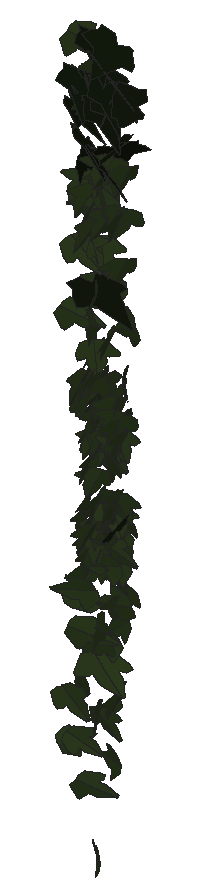
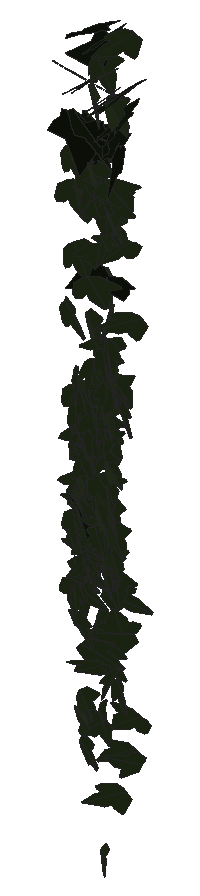
# SketchUp Ruby script. Lengths in inches.
U = 1.inch
M = Sketchup.active_model
def pt(a) = Geom::Point3d.new(a.map { |v| v * U })
def face(e, loops, mat)
  f = e.add_face(loops[0].map { |a| pt(a) })
  loops[1..].each { |l| e.add_face(l.map { |a| pt(a) }).erase! }
  f.material = f.back_material = mat if mat
  f
end
# faces: each face lists its corners as indices into pts; further lists are holes
def faces(e, pts, list, mat = nil) = list.each { |f| face(e, (f[0].is_a?(Array) ? f : [f]).map { |l| l.map { |i| pts[i] } }, mat) }
# xy, xz, yz: faces in a plane at the given z, y or x. An outline is a flat list of corners, or four numbers for a rectangle; further outlines are holes
def ring(l) = l.size == 4 ? [[l[0], l[1]], [l[2], l[1]], [l[2], l[3]], [l[0], l[3]]] : l.each_slice(2).to_a
def flat(e, list, mat, &to3) = list.each { |f| face(e, (f[0].is_a?(Array) ? f : [f]).map { |l| ring(l).map { |u, v| to3.(u, v) } }, mat) }
def xy(e, z, list, mat = nil) = flat(e, list, mat) { |x, y| [x, y, z] }
def xz(e, y, list, mat = nil) = flat(e, list, mat) { |x, z| [x, y, z] }
def yz(e, x, list, mat = nil) = flat(e, list, mat) { |y, z| [x, y, z] }
def lines(e, pts, list) = list.each { |a, b| e.add_line(pt(pts[a]), pt(pts[b])) }
# prism: a flat outline (further loops are holes) pulled along v
def prism(e, loops, v, mat = nil)
  f = face(e, loops, mat); d = Geom::Vector3d.new(v.map { |x| x * U })
  f.pushpull(f.normal.samedirection?(d) ? d.length : -d.length)
end
def box(e, o, s, mat = nil) = prism(e, [[o, [o[0] + s[0], o[1], o[2]], [o[0] + s[0], o[1] + s[1], o[2]], [o[0], o[1] + s[1], o[2]]]], [0, 0, s[2]], mat)
def at(x, y, z, deg = 0) = Geom::Transformation.translation(pt([x, y, z])) * Geom::Transformation.rotation(ORIGIN, Z_AXIS, deg.degrees)
def axes(o, x, y, z) = Geom::Transformation.new([*x, 0, *y, 0, *z, 0, *pt(o).to_a, 1])
def part(name) = M.definitions.add(name)
# library, detail: a bought-in or finely detailed component or shape, given as its bounding box
def library(name, o, s) = part(name).tap { |d| box(d.entities, o, s) }
def detail(e, o, s) = box(e.add_group.entities, o, s)
def put(e, d, t, mat = nil) = e.add_instance(d, t).tap { |i| i.material = mat if mat }
def group(e, t, mat = nil) = e.add_group.tap { |g| g.transformation = t; g.material = mat if mat }.entities
root = M.entities
M.materials.add("1026 AP 7946 SUNNY SIDE UP").color = [254, 231, 186]
M.materials.add("efeu1").color = [18, 25, 13]
M.materials.add("efeu2").color = [43, 57, 29]
c1 = part("ivyleaf_10")
p = [[0,0.5,-0.03],[-0.0625,2.02,-0.43],[-0.19,2.01,-0.46],[-0.54,1.05,-0.29],[-0.52,0.625,-0.18],[-0.83,0.76,-0.28],
  [-1.16,0.64,-0.33],[-1.15,0.33,-0.24],[-0.77,-0.39,0.02],[-0.3,-0.51,0.16],[0.04,-0.48,0.23],[-0.02,2.01,-0.4375],
  [-0.06,2.01,-0.43],[0.04,-0.49,0.23],[0.67,-0.49,0.14],[1.38,0.36,-0.2],[1.375,0.51,-0.24],[0.81,0.65,-0.19],
  [0.62,0.59,-0.15],[0.6,1.09,-0.28],[0.5,1.23,-0.31]]
faces(c1.entities,p,[[0,1,2,3,4,5,6,7,8,9,10],[11,12,0,13,14,15,16,17,18,19,20]],"efeu2")
c2 = part("ivyleaf_9")
p = [[1.54,2.16,1.25],[1.36,2.04,1.19],[-0.21,0.99,0.68],[-0.71,1.11,0.82],[-0.85,0.86,0.67],[-0.8,0.17,0.21],
  [-0.9,-0.01,0.1],[-0.67,-0.16,-0.02],[-0.08,-0.08,-0.05],[-0.03,-0.6,-0.4],[0.65,-0.88,-0.66],[0.83,-0.6,-0.49],
  [1.29,-0.42,-0.43],[1.8125,-0.07,-0.26],[1.21,0.44,0.15]]
faces(c2.entities,p,[[0,1,2,3,4,5,6,7,8,9,10,11,12,13,14]],"efeu1")
put(root,c1,axes([101.61,213.03,262.17],[0.23176,-0.14926,-0.08076],[-0.02073,0.09254,-0.20877],[0.26367,0.13847,0.05457]),"1026 AP 7946 SUNNY SIDE UP")
put(root,c2,axes([101.46,212.75,266.26],[0.24733,-0.16671,-0.10642],[-0.08833,0.08731,-0.23493],[0.29464,0.16612,0.0189]),"1026 AP 7946 SUNNY SIDE UP")
put(root,c1,axes([101.72,212.88,264.88],[-0.23689,-0.12528,0.14324],[-0.06836,-0.15104,-0.18865],[0.28709,-0.13934,0.07327]),"1026 AP 7946 SUNNY SIDE UP")
put(root,c1,axes([101.56,212.82,257.06],[0.27559,0.10864,-0.05443],[0.05387,0.0457,0.21169],[0.1826,-0.17745,0.0197]),"1026 AP 7946 SUNNY SIDE UP")
put(root,c2,axes([101.4375,213.02,266.65],[0.15677,-0.22108,-0.05738],[0.00234,0.06006,-0.24812],[0.35801,0.09642,0.02675]),"1026 AP 7946 SUNNY SIDE UP")
put(root,c1,axes([101.66,212.85,258.75],[-0.00671,-0.20722,0.02512],[-0.00265,-0.02553,-0.21367],[0.32829,-0.00444,-0.00121]),"1026 AP 7946 SUNNY SIDE UP")
put(root,c1,axes([101.59,212.96,256.3],[-0.03619,0.20773,0.06893],[-0.01152,0.06532,-0.21493],[-0.34241,-0.02415,-0.00006]),"1026 AP 7946 SUNNY SIDE UP")
put(root,c1,axes([101.86,212.6,257.48],[0.12653,0.00961,-0.2148],[-0.32827,0.006,-0.08266],[0.00337,0.22346,0.01276]),"1026 AP 7946 SUNNY SIDE UP")
put(root,c1,axes([101.42,212.63,255.43],[0.23805,0.04509,0.1535],[0.22598,0.03846,-0.16248],[-0.09307,0.20872,-0.0019]),"1026 AP 7946 SUNNY SIDE UP")
put(root,c1,axes([101.71,212.68,261],[0.22148,-0.18425,-0.10021],[-0.08169,0.08134,-0.23832],[0.31647,0.14994,0.00861]),"1026 AP 7946 SUNNY SIDE UP")
put(root,c1,axes([101.48,212.56,254.57],[0.08927,0.03452,-0.19843],[0.22167,0.13218,0.06791],[0.21384,-0.15142,0.01244]),"1026 AP 7946 SUNNY SIDE UP")
put(root,c2,axes([101.71,212.67,265.42],[0.07925,-0.05546,-0.25307],[-0.28866,0.16293,-0.07585],[0.27036,0.19022,-0.0068]),"1026 AP 7946 SUNNY SIDE UP")
put(root,c2,axes([101.54,212.87,266.64],[-0.03684,-0.24323,0.06027],[0.00647,-0.06051,-0.25189],[0.39382,-0.02176,0.00978]),"1026 AP 7946 SUNNY SIDE UP")
put(root,c1,axes([101.8125,212.59,255.85],[-0.14739,0.09172,0.16047],[-0.22078,0.07265,-0.13113],[-0.1779,-0.16616,0.02979]),"1026 AP 7946 SUNNY SIDE UP")
put(root,c1,axes([101.69,212.86,266.33],[0.04286,-0.2374,0.08742],[0.00963,-0.08606,-0.24665],[0.39701,0.02771,-0.00346]),"1026 AP 7946 SUNNY SIDE UP")
put(root,c1,axes([101.66,212.73,261.29],[0.01328,-0.20034,0.1191],[0.05041,-0.11469,-0.20582],[0.3611,0.02338,0.02435]),"1026 AP 7946 SUNNY SIDE UP")
put(root,c1,axes([101.72,212.88,261.76],[0.09502,-0.19344,-0.10823],[-0.02668,0.10339,-0.20774],[0.34427,0.0614,0.01377]),"1026 AP 7946 SUNNY SIDE UP")
put(root,c1,axes([101.47,212.64,262.49],[-0.11051,-0.10361,-0.20119],[0.30628,0.06671,-0.10861],[0.1627,-0.19596,0.0678]),"1026 AP 7946 SUNNY SIDE UP")
put(root,c1,axes([101.53,212.71,267.55],[-0.09663,-0.15585,-0.20096],[0.26263,0.12254,-0.15505],[0.29037,-0.1627,0.07336]),"1026 AP 7946 SUNNY SIDE UP")
put(root,c1,axes([101.73,212.83,258.35],[-0.01414,-0.20729,0.01577],[-0.00333,-0.0164,-0.21384],[0.32696,-0.00913,-0.0015]),"1026 AP 7946 SUNNY SIDE UP")
put(root,c1,axes([101.78,212.85,264.69],[-0.11994,-0.1968,0.11635],[-0.02853,-0.11465,-0.21697],[0.35653,-0.07538,0.02178]),"1026 AP 7946 SUNNY SIDE UP")
put(root,c1,axes([101.78,212.81,261.52],[0.09506,-0.21581,-0.0587],[-0.03511,0.05161,-0.23046],[0.34872,0.06403,-0.0072]),"1026 AP 7946 SUNNY SIDE UP")
put(root,c1,axes([101.77,212.69,257.78],[-0.1154,-0.18957,0.00063],[0.00594,-0.00327,-0.20938],[0.29803,-0.07334,0.00441]),"1026 AP 7946 SUNNY SIDE UP")
put(root,c1,axes([101.75,212.85,264.41],[0.14658,-0.22174,0.02744],[0.00316,-0.02939,-0.24778],[0.3514,0.09276,-0.00922]),"1026 AP 7946 SUNNY SIDE UP")
put(root,c1,axes([101.78,212.84,259.39],[0.1442,-0.18895,-0.06129],[-0.01091,0.06128,-0.21505],[0.31079,0.08982,0.02089]),"1026 AP 7946 SUNNY SIDE UP")
put(root,c1,axes([101.79,212.73,259.11],[0.03543,-0.20794,-0.03637],[0.00319,0.03453,-0.21519],[0.33133,0.0219,0.00596]),"1026 AP 7946 SUNNY SIDE UP")
put(root,c1,axes([101.79,212.88,264.54],[-0.26299,-0.16813,-0.00818],[0.03619,-0.0131,-0.24297],[0.26211,-0.16689,0.02534]),"1026 AP 7946 SUNNY SIDE UP")
put(root,c1,axes([101.82,212.78,264.08],[0.00136,-0.19115,0.14714],[0.01173,-0.14382,-0.19769],[0.37604,0.00518,0.00563]),"1026 AP 7946 SUNNY SIDE UP")
put(root,c1,axes([101.81,212.75,258.69],[-0.00967,-0.17007,-0.1392],[0.02296,0.13358,-0.17436],[0.33983,-0.01386,0.00782]),"1026 AP 7946 SUNNY SIDE UP")
put(root,c1,axes([101.8,212.88,258.02],[0.07527,-0.20039,-0.01726],[0.01418,0.01818,-0.21173],[0.31574,0.04696,0.01362]),"1026 AP 7946 SUNNY SIDE UP")
put(root,c1,axes([101.85,212.83,260.89],[0.0404,-0.21738,-0.05823],[-0.02444,0.05379,-0.225],[0.35184,0.0287,-0.00894]),"1026 AP 7946 SUNNY SIDE UP")
put(root,c1,axes([101.79,212.81,261.22],[-0.11763,-0.18359,-0.11534],[0.07918,0.09916,-0.20349],[0.32785,-0.08982,0.00776]),"1026 AP 7946 SUNNY SIDE UP")
put(root,c1,axes([101.85,212.86,261.83],[-0.05054,-0.22068,-0.04146],[0.0033,0.03909,-0.22949],[0.35236,-0.03202,-0.00379]),"1026 AP 7946 SUNNY SIDE UP")
put(root,c1,axes([101.84,212.98,259.08],[0.06676,-0.20368,0.01444],[-0.00351,-0.01596,-0.21436],[0.32113,0.04217,-0.00534]),"1026 AP 7946 SUNNY SIDE UP")
put(root,c1,axes([101.85,212.72,258.15],[-0.00269,-0.20464,0.01488],[0.00056,-0.01561,-0.21092],[0.32271,-0.00168,0.00049]),"1026 AP 7946 SUNNY SIDE UP")
put(root,c1,axes([101.86,212.66,258.57],[-0.03395,-0.19711,0.06331],[0.00278,-0.06309,-0.20447],[0.32517,-0.02004,0.00836]),"1026 AP 7946 SUNNY SIDE UP")
put(root,c1,axes([101.65,212.55,254.74],[0.11584,0.10359,0.16632],[0.17773,0.11551,-0.12928],[-0.24273,0.13401,-0.01529]),"1026 AP 7946 SUNNY SIDE UP")
put(root,c1,axes([101.84,212.74,259.83],[0.06507,-0.19625,0.0755],[0.01914,-0.07347,-0.20703],[0.32947,0.04303,-0.00289]),"1026 AP 7946 SUNNY SIDE UP")
put(root,c1,axes([101.88,212.92,267.09],[-0.05804,-0.24494,0.0506],[-0.00831,-0.05028,-0.25547],[0.39316,-0.03722,0.00207]),"1026 AP 7946 SUNNY SIDE UP")
put(root,c1,axes([101.66,212.625,263.79],[0.21552,0.17038,0.13839],[0.15447,0.09166,-0.22411],[-0.30313,0.16784,-0.01581]),"1026 AP 7946 SUNNY SIDE UP")
put(root,c1,axes([101.98,212.56,258.14],[0.23237,-0.0268,0.15395],[-0.22153,0.05408,0.15368],[-0.08961,-0.20321,0.0193]),"1026 AP 7946 SUNNY SIDE UP")
put(root,c1,axes([101.87,212.6875,261.42],[0.15944,-0.20959,0.04832],[0.0155,-0.04859,-0.23982],[0.33777,0.10116,-0.0118]),"1026 AP 7946 SUNNY SIDE UP")
put(root,c1,axes([101.98,212.74,256.53],[-0.30281,-0.02161,0.06658],[-0.09526,-0.03521,-0.19793],[0.04946,-0.2001,0.02642]),"1026 AP 7946 SUNNY SIDE UP")
put(root,c1,axes([101.875,212.74,260.44],[-0.05795,-0.18385,-0.11394],[0.05692,0.10421,-0.1921],[0.33167,-0.05001,0.01306]),"1026 AP 7946 SUNNY SIDE UP")
put(root,c1,axes([101.95,212.8125,259.55],[-0.16523,-0.16853,0.07901],[-0.0228,-0.08151,-0.20293],[0.29089,-0.10212,0.02898]),"1026 AP 7946 SUNNY SIDE UP")
put(root,c1,axes([102.04,212.67,258.04],[-0.2341,0.07876,0.1232],[-0.19245,0.01834,-0.16994],[-0.11574,-0.1898,0.03338]),"1026 AP 7946 SUNNY SIDE UP")
put(root,c1,axes([101.93,212.81,260.29],[-0.09309,-0.18076,0.11966],[0.00142,-0.12173,-0.19369],[0.33871,-0.04917,0.0337]),"1026 AP 7946 SUNNY SIDE UP")
put(root,c2,axes([101.69,212.79,265.61],[0.0999,-0.20559,0.13179],[0.07348,-0.12059,-0.22224],[0.37458,0.07848,0.00845]),"1026 AP 7946 SUNNY SIDE UP")
put(root,c1,axes([102.06,212.52,260.76],[0.01779,0.00664,0.24929],[-0.24562,0.18522,0.00337],[-0.29072,-0.15608,0.01241]),"1026 AP 7946 SUNNY SIDE UP")
put(root,c1,axes([102.13,212.86,256.53],[0.17523,-0.00808,-0.18643],[-0.28476,-0.00458,-0.11474],[0.00052,0.21244,-0.00832]),"1026 AP 7946 SUNNY SIDE UP")
put(root,c1,axes([101.99,212.86,260.65],[-0.25839,-0.14808,0.03879],[0.02039,-0.06976,-0.21986],[0.23972,-0.15368,0.0605]),"1026 AP 7946 SUNNY SIDE UP")
put(root,c1,axes([101.96,212.57,262.42],[0.08417,-0.12469,-0.19788],[0.02481,0.19811,-0.12727],[0.3583,0.01557,0.0553]),"1026 AP 7946 SUNNY SIDE UP")
put(root,c1,axes([101.99,212.89,258.64],[-0.20593,-0.15906,0.04633],[0.01478,-0.06555,-0.20687],[0.25988,-0.12231,0.04848]),"1026 AP 7946 SUNNY SIDE UP")
put(root,c1,axes([102,212.73,259.16],[0.00516,-0.21896,-0.01664],[-0.00853,0.01482,-0.22545],[0.34499,0.00364,-0.00532]),"1026 AP 7946 SUNNY SIDE UP")
put(root,c1,axes([102,212.73,260.74],[-0.04372,-0.20707,0.06584],[0.0083,-0.06624,-0.21518],[0.3412,-0.02492,0.01367]),"1026 AP 7946 SUNNY SIDE UP")
put(root,c1,axes([102.03,212.7,257.98],[0.23901,-0.13668,-0.06028],[-0.08348,0.02709,-0.20988],[0.21786,0.16033,-0.01428]),"1026 AP 7946 SUNNY SIDE UP")
put(root,c1,axes([102.06,212.9375,263.08],[-0.28105,-0.11279,0.09852],[-0.04045,-0.12491,-0.20068],[0.22963,-0.16004,0.08523]),"1026 AP 7946 SUNNY SIDE UP")
put(root,c1,axes([102.02,212.74,260.23],[0.12034,-0.20359,-0.05878],[-0.02602,0.05349,-0.22373],[0.33095,0.07824,0.00378]),"1026 AP 7946 SUNNY SIDE UP")
put(root,c1,axes([101.8,212.61,253.93],[-0.12831,-0.069,-0.19536],[0.27562,0.07626,-0.10607],[0.15603,-0.19145,0.02671]),"1026 AP 7946 SUNNY SIDE UP")
put(root,c1,axes([101.75,212.53,256.77],[-0.08837,-0.05138,-0.22728],[0.34744,0.03629,-0.06657],[0.0764,-0.22447,0.03985]),"1026 AP 7946 SUNNY SIDE UP")
put(root,c1,axes([102,212.9,260.79],[0.25946,-0.14821,-0.02505],[-0.00139,0.03393,-0.2269],[0.23594,0.16318,0.02621]),"1026 AP 7946 SUNNY SIDE UP")
put(root,c2,axes([101.87,212.85,267.46],[0.00623,-0.24228,0.07453],[0.02221,-0.07341,-0.24973],[0.39758,0.00789,0.01278]),"1026 AP 7946 SUNNY SIDE UP")
put(root,c1,axes([102.3,212.72,264.57],[-0.11422,0.04084,0.24101],[-0.37003,-0.04349,-0.06777],[0.04745,-0.24085,0.05161]),"1026 AP 7946 SUNNY SIDE UP")
put(root,c1,axes([102.07,212.52,263.03],[0.09753,-0.21119,-0.12507],[-0.0342,0.11874,-0.22578],[0.38057,0.06479,0.01176]),"1026 AP 7946 SUNNY SIDE UP")
put(root,c1,axes([102.05,212.73,261.45],[-0.00892,-0.22857,-0.0181],[0.00567,0.01619,-0.23543],[0.36027,-0.00592,0.00325]),"1026 AP 7946 SUNNY SIDE UP")
put(root,c1,axes([102.08,212.9375,265.08],[-0.14856,-0.21956,0.04773],[-0.01254,-0.04831,-0.24624],[0.35303,-0.09411,0.01134]),"1026 AP 7946 SUNNY SIDE UP")
put(root,c1,axes([102.03,212.82,260.4],[0.1169,-0.19681,-0.07919],[0.01795,0.08396,-0.21268],[0.33111,0.06493,0.03949]),"1026 AP 7946 SUNNY SIDE UP")
put(root,c1,axes([101.96,212.875,263.76],[0.15112,0.21359,-0.01638],[0.00054,-0.0189,-0.24126],[-0.33693,0.09577,-0.00773]),"1026 AP 7946 SUNNY SIDE UP")
put(root,c1,axes([101.96,212.67,261.96],[0.22067,0.17581,0.00542],[0.00176,0.00456,-0.23171],[-0.27652,0.14033,0.00285]),"1026 AP 7946 SUNNY SIDE UP")
put(root,c1,axes([102.01,212.875,261.17],[0.01761,-0.06828,0.21745],[0.05941,-0.20807,-0.07249],[0.34433,0.03939,0.00139]),"1026 AP 7946 SUNNY SIDE UP")
put(root,c1,axes([102.08,212.85,260.31],[-0.06056,-0.18967,0.11423],[-0.01453,-0.11217,-0.19969],[0.34602,-0.03791,0.01161]),"1026 AP 7946 SUNNY SIDE UP")
put(root,c1,axes([102.1,212.89,260.08],[-0.29149,-0.1159,0.01038],[-0.00162,-0.01855,-0.2248],[0.18302,-0.18476,0.01454]),"1026 AP 7946 SUNNY SIDE UP")
put(root,c1,axes([102.08,212.75,258.32],[0.08599,-0.1877,-0.06661],[0.00347,0.06654,-0.19999],[0.3116,0.05105,0.02061]),"1026 AP 7946 SUNNY SIDE UP")
put(root,c1,axes([102.16,212.5,252.67],[0.03993,-0.02687,-0.22204],[-0.08989,0.20837,-0.0325],[0.32924,0.06015,0.01805]),"1026 AP 7946 SUNNY SIDE UP")
put(root,c1,axes([102,212.73,255.35],[0.11166,-0.15546,0.11201],[0.10705,-0.08847,-0.17523],[0.27928,0.09606,0.02239]),"1026 AP 7946 SUNNY SIDE UP")
put(root,c1,axes([102.02,212.84,264.85],[0.0859,0.21342,0.11345],[-0.02046,0.11419,-0.22311],[-0.3762,0.04252,0.03804]),"1026 AP 7946 SUNNY SIDE UP")
put(root,c1,axes([102.08,212.81,264.52],[-0.22149,0.20765,0.06688],[0.05787,-0.05205,0.25819],[0.3366,0.14559,-0.00038]),"1026 AP 7946 SUNNY SIDE UP")
put(root,c1,axes([102.17,212.89,258.03],[0.13244,-0.12759,-0.14211],[-0.10554,0.11992,-0.15661],[0.27508,0.10744,0.00834]),"1026 AP 7946 SUNNY SIDE UP")
put(root,c1,axes([102.12,212.8125,266.41],[0.14272,-0.21997,-0.0798],[-0.02126,0.07668,-0.24414],[0.36543,0.09037,0.01696]),"1026 AP 7946 SUNNY SIDE UP")
put(root,c1,axes([101.99,212.73,260.23],[-0.23899,-0.10376,-0.11874],[0.17844,0.03439,-0.18682],[0.1652,-0.18726,0.03001]),"1026 AP 7946 SUNNY SIDE UP")
put(root,c1,axes([102.12,212.8,265.14],[0.07283,-0.24143,0.02037],[-0.00123,-0.02167,-0.25334],[0.38108,0.04607,-0.00471]),"1026 AP 7946 SUNNY SIDE UP")
put(root,c1,axes([102.15,212.89,260.17],[0.04057,-0.21524,-0.03032],[-0.01076,0.02759,-0.22314],[0.34117,0.02647,-0.00343]),"1026 AP 7946 SUNNY SIDE UP")
put(root,c2,axes([101.95,212.82,266.34],[0.09533,-0.24156,-0.02858],[-0.0027,0.02675,-0.25636],[0.38207,0.06046,0.00532]),"1026 AP 7946 SUNNY SIDE UP")
put(root,c1,axes([102.22,212.82,258.18],[-0.12431,-0.11695,-0.15566],[-0.161,-0.11129,0.14391],[-0.25269,0.12844,-0.01511]),"1026 AP 7946 SUNNY SIDE UP")
put(root,c1,axes([102.3,212.91,257.98],[0.20449,-0.05623,-0.17067],[-0.24969,0.04776,-0.14512],[0.11434,0.20488,-0.01166]),"1026 AP 7946 SUNNY SIDE UP")
put(root,c2,axes([101.93,212.96,266.82],[0.1178,-0.22427,-0.08363],[0.04143,0.09107,-0.23732],[0.37206,0.06087,0.05291]),"1026 AP 7946 SUNNY SIDE UP")
put(root,c1,axes([102.18,212.86,258.24],[0.22915,-0.10312,-0.10889],[-0.0848,0.10024,-0.17774],[0.21545,0.14913,0.04586]),"1026 AP 7946 SUNNY SIDE UP")
put(root,c1,axes([102.23,212.76,265.4],[-0.26105,-0.15088,0.09749],[-0.04607,-0.1056,-0.22499],[0.27696,-0.15978,0.05447]),"1026 AP 7946 SUNNY SIDE UP")
put(root,c1,axes([102.03,212.77,255.21],[-0.25652,0.04909,-0.12819],[0.17337,-0.06255,-0.17431],[-0.11981,-0.19559,0.02224]),"1026 AP 7946 SUNNY SIDE UP")
put(root,c1,axes([102.13,213,255.24],[0.16787,-0.1692,0.08506],[-0.04366,0.08084,0.20573],[-0.29348,-0.10881,0.01805]),"1026 AP 7946 SUNNY SIDE UP")
put(root,c1,axes([102.21,212.77,264.4375],[-0.05901,-0.1975,0.13998],[-0.0144,-0.13739,-0.20742],[0.37768,-0.0361,0.01397]),"1026 AP 7946 SUNNY SIDE UP")
put(root,c1,axes([102.17,212.65,259.01],[0.21498,-0.15409,-0.04625],[-0.01588,0.04946,-0.21039],[0.25148,0.13485,0.02625]),"1026 AP 7946 SUNNY SIDE UP")
put(root,c1,axes([102.23,212.84,260.97],[-0.10276,-0.20594,0.07272],[-0.00826,-0.0734,-0.22238],[0.34282,-0.0635,0.01644]),"1026 AP 7946 SUNNY SIDE UP")
put(root,c1,axes([102.12,212.82,259.99],[-0.1891,-0.15541,-0.12786],[0.14949,0.08131,-0.20075],[0.27371,-0.15178,0.02131]),"1026 AP 7946 SUNNY SIDE UP")
put(root,c1,axes([102.37,212.6,258.11],[0.16849,-0.02272,-0.1791],[-0.26059,0.05292,-0.11213],[0.08938,0.19713,0.01071]),"1026 AP 7946 SUNNY SIDE UP")
put(root,c2,axes([101.98,212.68,265.5],[0.25303,-0.18597,0.02259],[0.00404,-0.0281,-0.25295],[0.29462,0.16011,-0.01593]),"1026 AP 7946 SUNNY SIDE UP")
put(root,c1,axes([102.18,212.88,258.01],[-0.1794,0.16704,-0.00953],[-0.0053,-0.01464,-0.20816],[-0.26308,-0.11361,0.01069]),"1026 AP 7946 SUNNY SIDE UP")
put(root,c1,axes([102.21,212.68,261.4375],[-0.10872,-0.20562,-0.06766],[0.0626,0.05439,-0.22225],[0.33302,-0.07735,0.01969]),"1026 AP 7946 SUNNY SIDE UP")
put(root,c2,axes([101.98,212.64,263.13],[-0.06795,-0.10476,-0.23824],[0.27861,0.15474,-0.1057],[0.2847,-0.17643,0.04657]),"1026 AP 7946 SUNNY SIDE UP")
put(root,c1,axes([102.45,212.9,258.38],[-0.03372,0.05887,0.19957],[-0.31647,0.01197,-0.02668],[-0.02972,-0.1942,0.05761]),"1026 AP 7946 SUNNY SIDE UP")
put(root,c1,axes([102.21,212.47,256.97],[0.0431,-0.14797,-0.18783],[0.05822,0.18316,-0.14702],[0.36357,-0.01179,0.04581]),"1026 AP 7946 SUNNY SIDE UP")
put(root,c1,axes([102.03,212.74,256.19],[-0.32337,-0.15609,-0.10367],[0.30516,-0.13615,-0.14863],[0.05459,-0.16351,0.21677]),"1026 AP 7946 SUNNY SIDE UP")
put(root,c1,axes([102.26,212.69,262.25],[0.08799,-0.23075,-0.00798],[-0.00913,0.00522,-0.24453],[0.36285,0.05608,-0.00422]),"1026 AP 7946 SUNNY SIDE UP")
put(root,c1,axes([102.24,212.82,260.28],[-0.05055,-0.15007,0.16269],[0.04692,-0.16199,-0.15246],[0.3403,0.00004,0.04519]),"1026 AP 7946 SUNNY SIDE UP")
put(root,c2,axes([102.1,212.82,266.71],[0.04606,-0.25044,0.005],[-0.00027,-0.00634,-0.2598],[0.39392,0.02928,-0.00077]),"1026 AP 7946 SUNNY SIDE UP")
put(root,c2,axes([102.25,212.87,267.52],[-0.2007,-0.19649,0.10538],[-0.03846,-0.10611,-0.23943],[0.34701,-0.1254,0.03441]),"1026 AP 7946 SUNNY SIDE UP")
put(root,c1,axes([102.23,212.68,258.82],[-0.00786,-0.03271,-0.22447],[0.06945,0.21318,-0.03279],[0.33912,-0.04441,0.00151]),"1026 AP 7946 SUNNY SIDE UP")
put(root,c1,axes([102.1875,212.89,258.11],[-0.01597,-0.11925,-0.17673],[0.12922,0.15492,-0.1155],[0.30108,-0.07281,0.04019]),"1026 AP 7946 SUNNY SIDE UP")
put(root,c2,axes([102,212.73,267.14],[0.25611,-0.17674,0.08852],[0.06649,-0.07879,-0.24712],[0.30248,0.16696,-0.02063]),"1026 AP 7946 SUNNY SIDE UP")
put(root,c1,axes([102.39,213,258.83],[-0.22772,0.11952,0.12997],[-0.17769,0.05884,-0.19176],[-0.20658,-0.18237,0.02167]),"1026 AP 7946 SUNNY SIDE UP")
put(root,c2,axes([102.44,212.67,265.78],[-0.16099,0.22903,-0.01518],[-0.00433,-0.01878,-0.25835],[-0.36099,-0.10192,0.00986]),"1026 AP 7946 SUNNY SIDE UP")
put(root,c1,axes([102.29,212.82,260.21],[-0.05839,-0.21175,0.03532],[0.03306,-0.03943,-0.21993],[0.33599,-0.03292,0.02778]),"1026 AP 7946 SUNNY SIDE UP")
put(root,c1,axes([102.32,212.58,260.08],[-0.26579,0.13099,0.04557],[-0.06377,0.01859,-0.21996],[-0.20745,-0.17355,0.00923]),"1026 AP 7946 SUNNY SIDE UP")
put(root,c1,axes([102.24,212.77,258.57],[-0.17868,-0.15002,-0.10563],[0.11381,0.07246,-0.19305],[0.26126,-0.13417,0.01185]),"1026 AP 7946 SUNNY SIDE UP")
put(root,c1,axes([102.3125,212.8,255.57],[-0.00294,-0.20087,0.02984],[0.00083,-0.03012,-0.20712],[0.31938,-0.00177,0.00082]),"1026 AP 7946 SUNNY SIDE UP")
put(root,c1,axes([102.38,212.93,261.36],[-0.12029,0.16265,0.1362],[-0.16218,0.09222,-0.17908],[-0.28587,-0.12076,0.04429]),"1026 AP 7946 SUNNY SIDE UP")
put(root,c1,axes([102.25,212.89,260.32],[-0.26942,-0.12531,-0.05247],[0.11206,-0.01503,-0.21192],[0.18028,-0.17792,0.0533]),"1026 AP 7946 SUNNY SIDE UP")
put(root,c1,axes([102.35,212.8125,260.58],[-0.02434,-0.21813,0.02905],[-0.00078,-0.02947,-0.22545],[0.3461,-0.0154,0.00153]),"1026 AP 7946 SUNNY SIDE UP")
put(root,c1,axes([102.35,212.91,260.72],[-0.05324,-0.21948,0.00587],[0.00586,-0.0076,-0.22877],[0.34523,-0.03372,0.00479]),"1026 AP 7946 SUNNY SIDE UP")
put(root,c2,axes([102.35,212.73,265.73],[0.17715,0.23317,-0.04247],[-0.01842,-0.04157,-0.26691],[-0.37223,0.11302,-0.007]),"1026 AP 7946 SUNNY SIDE UP")
put(root,c1,axes([102.47,212.58,254.54],[0.06559,-0.05816,-0.20491],[-0.17432,0.16475,-0.07274],[0.27471,0.11843,0.00276]),"1026 AP 7946 SUNNY SIDE UP")
put(root,c1,axes([102.36,212.88,260.37],[-0.09383,0.21024,0.03113],[-0.09839,0.01138,-0.21739],[-0.31887,-0.06537,0.05792]),"1026 AP 7946 SUNNY SIDE UP")
put(root,c1,axes([102.42,212.84,256.98],[0.20946,-0.12033,-0.12144],[-0.13397,0.0805,-0.18445],[0.22762,0.15811,0.00318]),"1026 AP 7946 SUNNY SIDE UP")
put(root,c1,axes([102.33,212.88,260.6],[0.04176,-0.21724,-0.033],[0.03265,0.03337,-0.22386],[0.34345,0.02324,0.0253]),"1026 AP 7946 SUNNY SIDE UP")
put(root,c1,axes([102.58,212.68,257.41],[-0.11014,0.01921,0.21662],[-0.33072,-0.02453,-0.07005],[0.02723,-0.22017,0.02539]),"1026 AP 7946 SUNNY SIDE UP")
put(root,c1,axes([102.34,212.86,261.11],[0.14477,-0.20729,-0.01868],[-0.00173,0.01805,-0.23347],[0.32702,0.09186,0.00703]),"1026 AP 7946 SUNNY SIDE UP")
put(root,c1,axes([102.26,212.93,259.12],[0.30556,-0.08049,0.06032],[0.07051,-0.04496,-0.2156],[0.1402,0.19805,-0.02303]),"1026 AP 7946 SUNNY SIDE UP")
put(root,c1,axes([102.39,212.87,263.55],[-0.13295,-0.21659,0.04788],[-0.01077,-0.04848,-0.23954],[0.34856,-0.08411,0.01086]),"1026 AP 7946 SUNNY SIDE UP")
put(root,c2,axes([102.49,212.56,258.81],[-0.02226,0.18552,0.16261],[-0.01344,0.15658,-0.19074],[-0.3817,-0.01634,-0.00277]),"1026 AP 7946 SUNNY SIDE UP")
put(root,c1,axes([102.44,212.93,257.55],[-0.27107,0.09888,0.04419],[-0.08827,-0.01449,-0.20072],[-0.14427,-0.17692,0.03977]),"1026 AP 7946 SUNNY SIDE UP")
put(root,c1,axes([102.39,212.8125,259.21],[0.05127,-0.18325,0.10384],[0.01393,-0.10177,-0.19217],[0.32936,0.03283,-0.00804]),"1026 AP 7946 SUNNY SIDE UP")
put(root,c1,axes([102.59,212.875,262.4375],[-0.14,0.0875,0.19691],[-0.29426,0.06043,-0.11825],[-0.149,-0.20155,0.04852]),"1026 AP 7946 SUNNY SIDE UP")
put(root,c1,axes([102.41,212.77,257.44],[-0.06214,-0.20691,-0.002],[0.00443,0.00024,-0.21699],[0.32531,-0.03953,0.00257]),"1026 AP 7946 SUNNY SIDE UP")
put(root,c1,axes([102.17,212.81,258.31],[-0.11669,0.00653,-0.19967],[0.28018,-0.07971,-0.0735],[-0.12049,-0.19166,0.02245]),"1026 AP 7946 SUNNY SIDE UP")
put(root,c1,axes([102.27,212.75,259.04],[0.29104,0.08371,0.0664],[0.10271,0.01031,-0.20851],[-0.12999,0.19557,-0.01608]),"1026 AP 7946 SUNNY SIDE UP")
put(root,c1,axes([102.4,212.57,259.21],[0.03457,-0.19606,-0.0845],[0.03298,0.08296,-0.20072],[0.33187,0.01218,0.02875]),"1026 AP 7946 SUNNY SIDE UP")
put(root,c1,axes([102.43,212.82,260.41],[0.03945,-0.21032,0.0739],[0.00909,-0.07275,-0.21861],[0.3499,0.0256,-0.00265]),"1026 AP 7946 SUNNY SIDE UP")
put(root,c1,axes([102.46,212.88,265.27],[-0.0876,-0.23459,0.05867],[-0.00719,-0.05878,-0.24857],[0.38001,-0.05519,0.00882]),"1026 AP 7946 SUNNY SIDE UP")
put(root,c1,axes([102.43,212.68,259.39],[0.04844,-0.18439,0.11],[0.01564,-0.10758,-0.19309],[0.3355,0.03164,-0.00688]),"1026 AP 7946 SUNNY SIDE UP")
put(root,c1,axes([102.51,212.76,264.57],[-0.28993,-0.13937,0.05983],[-0.05052,-0.05462,-0.2372],[0.23247,-0.18569,0.02308]),"1026 AP 7946 SUNNY SIDE UP")
put(root,c1,axes([102.38,212.72,259.33],[-0.33234,-0.00993,-0.06744],[0.10374,-0.0156,-0.21729],[0.00762,-0.2207,0.0171]),"1026 AP 7946 SUNNY SIDE UP")
put(root,c1,axes([102.54,212.64,260.87],[-0.25841,-0.11905,0.08796],[-0.09288,-0.06468,-0.20876],[0.21149,-0.17387,0.01579]),"1026 AP 7946 SUNNY SIDE UP")
put(root,c1,axes([102.47,212.66,260.75],[-0.07827,-0.21479,-0.00114],[0.00425,-0.00074,-0.22713],[0.33771,-0.04977,0.00259]),"1026 AP 7946 SUNNY SIDE UP")
put(root,c2,axes([102.73,212.74,266.62],[-0.32836,0.12036,0.08715],[-0.16873,-0.02575,-0.23722],[-0.15733,-0.22358,0.07253]),"1026 AP 7946 SUNNY SIDE UP")
put(root,c1,axes([102.47,212.65,264.54],[0.04002,-0.24274,-0.01229],[-0.00206,0.01047,-0.25138],[0.38204,0.02549,-0.00007]),"1026 AP 7946 SUNNY SIDE UP")
